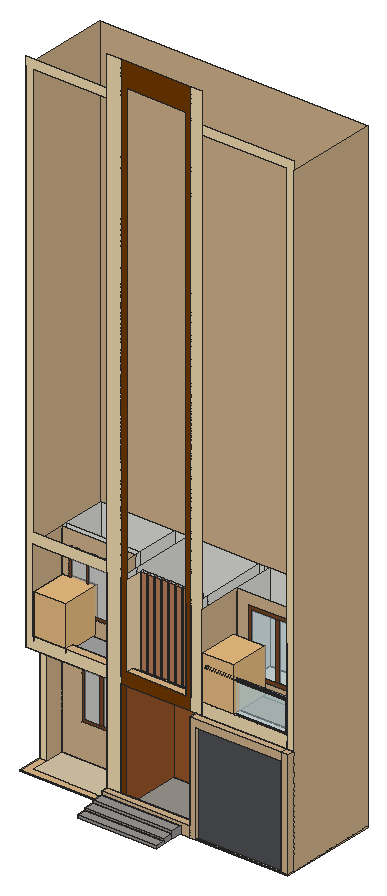
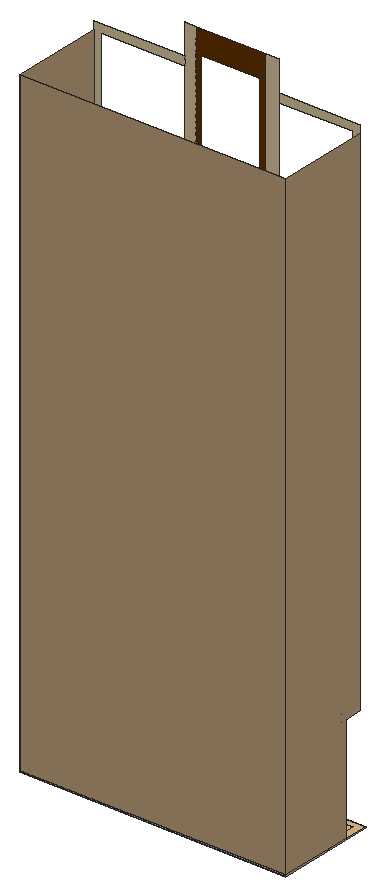
# SketchUp Ruby script. Lengths in inches.
U = 1.inch
M = Sketchup.active_model
def pt(a) = Geom::Point3d.new(a.map { |v| v * U })
def face(e, loops, mat)
  f = e.add_face(loops[0].map { |a| pt(a) })
  loops[1..].each { |l| e.add_face(l.map { |a| pt(a) }).erase! }
  f.material = f.back_material = mat if mat
  f
end
# faces: each face lists its corners as indices into pts; further lists are holes
def faces(e, pts, list, mat = nil) = list.each { |f| face(e, (f[0].is_a?(Array) ? f : [f]).map { |l| l.map { |i| pts[i] } }, mat) }
# xy, xz, yz: faces in a plane at the given z, y or x. An outline is a flat list of corners, or four numbers for a rectangle; further outlines are holes
def ring(l) = l.size == 4 ? [[l[0], l[1]], [l[2], l[1]], [l[2], l[3]], [l[0], l[3]]] : l.each_slice(2).to_a
def flat(e, list, mat, &to3) = list.each { |f| face(e, (f[0].is_a?(Array) ? f : [f]).map { |l| ring(l).map { |u, v| to3.(u, v) } }, mat) }
def xy(e, z, list, mat = nil) = flat(e, list, mat) { |x, y| [x, y, z] }
def xz(e, y, list, mat = nil) = flat(e, list, mat) { |x, z| [x, y, z] }
def yz(e, x, list, mat = nil) = flat(e, list, mat) { |y, z| [x, y, z] }
def lines(e, pts, list) = list.each { |a, b| e.add_line(pt(pts[a]), pt(pts[b])) }
# prism: a flat outline (further loops are holes) pulled along v
def prism(e, loops, v, mat = nil)
  f = face(e, loops, mat); d = Geom::Vector3d.new(v.map { |x| x * U })
  f.pushpull(f.normal.samedirection?(d) ? d.length : -d.length)
end
def box(e, o, s, mat = nil) = prism(e, [[o, [o[0] + s[0], o[1], o[2]], [o[0] + s[0], o[1] + s[1], o[2]], [o[0], o[1] + s[1], o[2]]]], [0, 0, s[2]], mat)
def at(x, y, z, deg = 0) = Geom::Transformation.translation(pt([x, y, z])) * Geom::Transformation.rotation(ORIGIN, Z_AXIS, deg.degrees)
def axes(o, x, y, z) = Geom::Transformation.new([*x, 0, *y, 0, *z, 0, *pt(o).to_a, 1])
def part(name) = M.definitions.add(name)
# library, detail: a bought-in or finely detailed component or shape, given as its bounding box
def library(name, o, s) = part(name).tap { |d| box(d.entities, o, s) }
def detail(e, o, s) = box(e.add_group.entities, o, s)
def put(e, d, t, mat = nil) = e.add_instance(d, t).tap { |i| i.material = mat if mat }
def group(e, t, mat = nil) = e.add_group.tap { |g| g.transformation = t; g.material = mat if mat }.entities
root = M.entities
M.materials.add("[0034_Wheat]").color = [245, 222, 179]
M.materials.add("[0035_Tan]").color = [210, 180, 140]
M.materials.add("[0036_BurlyWood]1").color = [222, 184, 135]
M.materials.add("[Blinds Roman Hobbled Blue]").color = [81, 82, 87]
M.materials.add("[Carpet Berber Pattern Gray]").color = [165, 165, 165]
M.materials.add("[Color C07]").color = [114, 57, 0]
M.materials.add("[Concrete Aggregate Smoke]").color = [154, 150, 148]
M.materials.add("[Field Square Tile]").color = [217, 201, 169]
M.materials.add("[Formica Beige]").color = [247, 219, 174]
M.materials.add("[Formica Laminate Dark]").color = [50, 53, 60]
M.materials.add("[Granite Tile]").color = [155, 148, 143]
M.materials.add("[Tile Veriegated Stone]").color = [171, 137, 112]
M.materials.add("[Translucent Glass Gray]").color = [191, 191, 191]
M.materials["[Translucent Glass Gray]"].alpha = 0.5
M.materials.add("[Translucent Glass Safety]").color = [204, 235, 244]
M.materials["[Translucent Glass Safety]"].alpha = 0.5
M.materials.add("[Wood Cherry Original]1").color = [152, 86, 42]
M.materials.add("[Wood Veneer 01]").color = [120, 70, 37]
M.materials.add("[Wood Veneer 02]").color = [190, 128, 91]
c1 = library("chau cay",[-24.34,-109.24,0],[56.46,62.58,79.69])
xy(root,0,[[646.67,0,1274.49,73.07],[646.67,73.07,1274.49,155.22],[646.67,155.22,1274.49,237.375],[0,237.375,2128.29,1030.11]])
xy(root,9,[[2069.85,237.375,2128.29,295.82],[1398.32,257.25,2069.85,283.5625],[2069.85,295.82,2069.85,971.67,58.44,971.67,58.44,433.5,0,433.5,0,1030.11,2128.29,1030.11,2128.29,295.82],[646.67,295.82,646.67,971.67,726.78,971.67,726.78,763.98,752.97,763.98,752.97,295.82],[752.97,295.82,800.41,763.98],
  [1351.23,295.82,1398.32,971.67],[1398.32,295.82,2069.85,971.67],[58.44,584.29,646.67,971.67],[726.78,763.98,1351.23,971.67]])
xy(root,9,[[0,237.375,646.67,237.375,646.67,295.82,58.44,295.82,58.44,433.5,0,433.5],[1398.32,237.375,2069.85,257.25]],"[0036_BurlyWood]1")
xy(root,9,[[58.44,295.82,646.67,584.29]],"[Field Square Tile]")
xy(root,9,[[800.41,295.82,1351.23,763.98]],"[Granite Tile]")
xy(root,22.375,[[646.67,0,1274.49,73.07]],"[Concrete Aggregate Smoke]")
xy(root,39.375,[[646.67,73.07,1274.49,155.22]],"[Concrete Aggregate Smoke]")
xy(root,58.875,[[646.67,155.22,1274.49,237.375]],"[Concrete Aggregate Smoke]")
xy(root,86.125,[[646.67,237.375,1351.23,295.82]],"[0035_Tan]")
xy(root,800.1875,[[1398.32,237.375,2069.85,257.25]],"[0036_BurlyWood]1")
xy(root,862.75,[[752.97,295.82,800.41,584.29],[1351.23,295.82,1398.32,584.29],[1398.32,295.82,2069.85,584.29],[58.44,584.29,646.67,971.67],[646.67,584.29,646.67,971.67,726.78,971.67,726.78,763.98,752.97,763.98,752.97,584.29],
  [752.97,584.29,800.41,763.98],[1351.23,584.29,1398.32,971.67],[1398.32,584.29,2069.85,971.67],[726.78,763.98,1351.23,971.67]])
xy(root,862.75,[[1351.23,237.375,2069.85,295.82],[2069.85,237.375,2128.29,295.82],[0,295.82,0,433.5,58.44,433.5,58.44,584.29,646.67,584.29,646.67,295.82]],"[0035_Tan]")
xy(root,862.75,[[800.41,295.82,1351.23,584.29],[800.41,584.29,1351.23,763.98]],"[Wood Cherry Original]1")
xy(root,918.8125,[[752.97,358.94,800.41,457.98],[1272.8,358.94,1313.62,457.98],[1313.62,358.94,1398.32,971.67],[800.41,433.79,848.4,457.98],[856.53,433.79,904.52,457.98],
  [912.66,433.79,960.65,457.98],[968.78,433.79,1016.77,457.98],[1024.91,433.79,1072.9,457.98],[1081.03,433.79,1129.02,457.98],[1137.16,433.79,1185.15,457.98],
  [1192.22,433.79,1232.95,457.98],[1240.21,433.79,1272.8,457.98],[752.97,457.98,1313.62,971.67],[58.44,584.29,646.67,623.89],[58.44,623.89,646.67,971.67],
  [1398.32,647.48,2069.85,971.67]])
xy(root,918.8125,[[800.41,358.94,1272.8,358.94,1272.8,433.79,1240.21,433.79,1240.21,457.98,1232.95,457.98,1232.95,433.79,1192.22,433.79,1192.22,457.98,1185.15,457.98,1185.15,433.79,1137.16,433.79,1137.16,457.98,1129.02,457.98,1129.02,433.79,1081.03,433.79,1081.03,457.98,1072.9,457.98,1072.9,433.79,1024.91,433.79,1024.91,457.98,1016.77,457.98,1016.77,433.79,968.78,433.79,968.78,457.98,960.65,457.98,960.65,433.79,912.66,433.79,912.66,457.98,904.52,457.98,904.52,433.79,856.53,433.79,856.53,457.98,848.4,457.98,848.4,433.79,800.41,433.79]],"[0036_BurlyWood]1")
xy(root,918.8125,[[58.44,358.94,646.67,584.29]],"[Carpet Berber Pattern Gray]")
xy(root,918.8125,[[1398.32,358.94,2069.85,647.48]],"[Tile Veriegated Stone]")
xy(root,961.5625,[[1414.96,312.46,2052.74,358.94],[1407.92,319.86,1406.26,319.88,1404.65,320.34,1403.23,321.19,1402.07,322.39,1401.26,323.84,1400.85,325.45,1400.875,327.12,1401.33,328.72,1402.18,330.15,1403.375,331.31,1404.83,332.12,1406.44,332.52,1408.11,332.5,1409.71,332.04,1411.14,331.19,1412.3,330,1413.11,328.54,1413.51,326.93,1413.49,325.27,1413.03,323.66,1412.18,322.24,1410.99,321.08,1409.53,320.27],[2060.17,319.86,2058.51,319.88,2056.9,320.34,2055.48,321.19,2054.32,322.39,2053.51,323.84,2053.1,325.45,2053.125,327.12,2053.58,328.72,2054.43,330.15,2055.625,331.31,2057.08,332.12,2058.69,332.52,2060.36,332.5,2061.96,332.04,2063.39,331.19,2064.55,330,2065.36,328.54,2065.76,326.93,2065.74,325.27,2065.28,323.66,2064.43,322.24,2063.24,321.08,2061.78,320.27]])
xy(root,961.5625,[[1398.32,295.82,2052.74,312.46],[2052.74,295.82,2069.85,312.46],[[1398.32,312.46,1414.96,358.94],[1407.92,319.86,1406.26,319.88,1404.65,320.34,1403.23,321.19,1402.07,322.39,1401.26,323.84,1400.85,325.45,1400.875,327.12,1401.33,328.72,1402.18,330.15,1403.375,331.31,1404.83,332.12,1406.44,332.52,1408.11,332.5,1409.71,332.04,1411.14,331.19,1412.3,330,1413.11,328.54,1413.51,326.93,1413.49,325.27,1413.03,323.66,1412.18,322.24,1410.99,321.08,1409.53,320.27]],[[2052.74,312.46,2069.85,358.94],[2060.17,319.86,2058.51,319.88,2056.9,320.34,2055.48,321.19,2054.32,322.39,2053.51,323.84,2053.1,325.45,2053.125,327.12,2053.58,328.72,2054.43,330.15,2055.625,331.31,2057.08,332.12,2058.69,332.52,2060.36,332.5,2061.96,332.04,2063.39,331.19,2064.55,330,2065.36,328.54,2065.76,326.93,2065.74,325.27,2065.28,323.66,2064.43,322.24,2063.24,321.08,2061.78,320.27]]],"[0034_Wheat]")
xy(root,961.5625,[[58.44,295.82,646.67,358.94],[800.41,295.82,1272.8,358.94]],"[0036_BurlyWood]1")
xy(root,1187.43,[[1414.96,312.46,2052.74,358.94]],"[Translucent Glass Safety]")
xy(root,1192.93,[[1407.92,319.86,1408.5,320.01,1405.82,320.01,1406.26,319.88],[1405.82,320.01,1408.5,320.01,1409.53,320.27,1410.99,321.08,1412.18,322.24,1413.03,323.66,1413.49,325.27,1413.51,326.93,1413.11,328.54,1412.3,330,1411.14,331.19,1409.71,332.04,1408.11,332.5,1406.44,332.52,1404.83,332.12,1403.375,331.31,1402.18,330.15,1401.33,328.72,1400.875,327.12,1400.85,325.45,1401.26,323.84,1402.07,322.39,1403.23,321.19,1404.65,320.34]])
xy(root,1193.4375,[[2060.17,319.86,2061.78,320.27,2063.24,321.08,2064.43,322.24,2065.28,323.66,2065.74,325.27,2065.76,326.93,2065.36,328.54,2064.55,330,2063.39,331.19,2061.96,332.04,2060.36,332.5,2058.69,332.52,2057.08,332.12,2055.625,331.31,2054.43,330.15,2053.58,328.72,2053.125,327.12,2053.1,325.45,2053.51,323.84,2054.32,322.39,2055.48,321.19,2056.9,320.34,2058.51,319.88]])
xz(root,0,[[646.67,0,1274.49,22.375]],"[Concrete Aggregate Smoke]")
xz(root,73.07,[[646.67,0,1274.49,22.375]])
xz(root,73.07,[[646.67,22.375,1274.49,39.375]],"[Concrete Aggregate Smoke]")
xz(root,155.22,[[646.67,0,1274.49,39.375]])
xz(root,155.22,[[646.67,39.375,1274.49,58.875]],"[Concrete Aggregate Smoke]")
xz(root,237.375,[[646.67,0,1274.49,58.875]])
xz(root,237.375,[[1274.49,0,1351.23,0,1351.23,86.125,646.67,86.125,646.67,58.875,1274.49,58.875],[1351.23,0,1398.32,0,1398.32,800.1875,2069.85,800.1875,2069.85,862.75,1351.23,862.75],[2069.85,9,2128.29,862.75]],"[0035_Tan]")
xz(root,237.375,[[0,0,646.67,9],[1398.32,0,2128.29,9]],"[0036_BurlyWood]1")
xz(root,257.25,[[1398.32,9,2069.85,800.1875]],"[Blinds Roman Hobbled Blue]")
xz(root,295.82,[[646.67,9,752.97,86.125],[752.97,9,800.41,86.125],[1351.23,9,1398.32,862.75],[1398.32,9,2069.85,862.75],[2069.85,9,2128.29,862.75]])
xz(root,295.82,[[646.67,86.125,752.97,5306.25],[0,862.75,646.67,862.75,646.67,961.5625,58.44,961.5625,58.44,1615.875,646.67,1615.875,646.67,1695.75,58.44,1695.75,58.44,4996.25,646.67,4996.25,646.67,5063.875,0,5063.875],[1313.62,862.75,1398.32,5306.25],[1398.32,862.75,2069.85,961.5625],[2069.85,862.75,2128.29,862.75,2128.29,5063.875,1398.32,5063.875,1398.32,4996.25,2069.85,4996.25]],"[0034_Wheat]")
xz(root,295.82,[[800.41,9,1351.23,86.125]],"[0035_Tan]")
xz(root,295.82,[[752.97,86.125,800.41,862.75],[[752.97,862.75,1313.62,5306.25],[800.41,961.5625,1272.8,5116.2]]],"[Color C07]")
xz(root,312.46,[[1414.96,961.5625,2052.74,1187.43]],"[Translucent Glass Safety]")
xz(root,358.94,[[58.44,918.8125,646.67,961.5625],[1272.8,918.8125,1313.62,961.5625],[1313.62,918.8125,1398.32,961.5625],[1398.32,918.8125,2069.85,961.5625]])
xz(root,358.94,[[800.41,918.8125,1272.8,961.5625]],"[0036_BurlyWood]1")
xz(root,358.94,[[1414.96,961.5625,2052.74,1187.43]],"[Translucent Glass Safety]")
xz(root,433.5,[[0,9,58.44,862.75]],"[0034_Wheat]")
xz(root,433.79,[[800.41,918.8125,848.4,1615.875],[856.53,918.8125,904.52,1615.875],[912.66,918.8125,960.65,1615.875],[968.78,918.8125,1016.77,1615.875],[1024.91,918.8125,1072.9,1615.875],
  [1081.03,918.8125,1129.02,1615.875],[1137.16,918.8125,1185.15,1615.875],[1192.22,918.8125,1232.95,1615.875],[1240.21,918.8125,1272.8,1615.875]],"[Wood Veneer 02]")
xz(root,457.98,[[800.41,918.8125,848.4,1615.875],[856.53,918.8125,904.52,1615.875],[912.66,918.8125,960.65,1615.875],[968.78,918.8125,1016.77,1615.875],[1024.91,918.8125,1072.9,1615.875],
  [1081.03,918.8125,1129.02,1615.875],[1137.16,918.8125,1185.15,1615.875],[1192.22,918.8125,1232.95,1615.875],[1240.21,918.8125,1272.8,1615.875]])
xz(root,457.98,[[848.4,918.8125,856.53,1615.875],[904.52,918.8125,912.66,1615.875],[960.65,918.8125,968.78,1615.875],[1016.77,918.8125,1024.91,1615.875],[1072.9,918.8125,1081.03,1615.875],
  [1129.02,918.8125,1137.16,1615.875],[1185.15,918.8125,1192.22,1615.875],[1232.95,918.8125,1240.21,1615.875]],"[Formica Laminate Dark]")
xz(root,584.29,[[[58.44,9,646.67,862.75],[211.5625,275.46,542.4375,741.34]],[[58.44,918.8125,646.67,1615.875],[113.6,1037.93,575.6,1499.93]]],"[0035_Tan]")
xz(root,584.29,[[234.18,298.08,360.07,718.72],[385.8125,298.08,519.82,718.72],[133.43,1057.76,252.99,1480.1],[266.84,1057.76,428.61,1480.1],[442.47,1057.76,555.77,1480.1]],"[Translucent Glass Gray]")
xz(root,584.29,[[[211.5625,275.46,542.4375,741.34],[234.18,298.08,519.82,718.72]],[360.07,298.08,385.8125,718.72],[[113.6,1037.93,575.6,1499.93],[133.43,1057.76,555.77,1480.1]],[252.99,1057.76,266.84,1480.1],[428.61,1057.76,442.47,1480.1]],"[Wood Veneer 01]")
xz(root,623.89,[[58.44,918.8125,646.67,1615.875]])
xz(root,647.48,[[[1398.32,918.8125,2069.85,1615.875],[1485.05,1017.34,1964.11,1534.78]]],"[0035_Tan]")
xz(root,647.48,[[1515.31,1047.6,1702.55,1504.52],[1732.8,1047.6,1933.85,1504.52]],"[Translucent Glass Safety]")
xz(root,647.48,[[[1485.05,1017.34,1964.11,1534.78],[1515.31,1047.6,1933.85,1504.52]],[1702.55,1047.6,1732.8,1504.52]],"[Wood Veneer 01]")
xz(root,763.98,[[726.78,9,752.97,862.75],[752.97,9,800.41,862.75]])
xz(root,763.98,[[800.41,9,1351.23,862.75]],"[Wood Cherry Original]1")
xz(root,971.67,[[58.44,9,646.67,862.75],[646.67,9,726.78,862.75],[726.78,9,1351.23,862.75],[1351.23,9,1398.32,862.75],[1398.32,9,2069.85,862.75],
  [58.44,862.75,646.67,918.8125],[646.67,862.75,726.78,918.8125],[726.78,862.75,1351.23,918.8125],[1351.23,862.75,1398.32,918.8125],[1398.32,862.75,2069.85,918.8125],
  [58.44,918.8125,646.67,1615.875],[646.67,918.8125,726.78,1615.875],[726.78,918.8125,752.97,1615.875],[752.97,918.8125,1313.62,1615.875],[1313.62,918.8125,1351.23,1615.875],
  [1351.23,918.8125,1398.32,1615.875],[1398.32,918.8125,2069.85,1615.875]])
xz(root,1030.11,[[0,0,2128.29,9]])
xz(root,1030.11,[[0,9,2128.29,4996.25]],"[0035_Tan]")
yz(root,0,[[433.5,9,433.5,862.75,295.82,862.75,295.82,4996.25,1030.11,4996.25,1030.11,9]],"[0035_Tan]")
yz(root,0,[[237.375,0,1030.11,9]],"[0036_BurlyWood]1")
yz(root,58.44,[[584.29,9,971.67,862.75],[481.57,862.75,584.29,918.8125],[584.29,862.75,971.67,918.8125],[584.29,918.8125,623.89,1615.875],[623.89,918.8125,971.67,1615.875]])
yz(root,58.44,[[433.5,9,584.29,862.75],[358.94,918.8125,584.29,918.8125,584.29,1615.875,295.82,1615.875,295.82,961.5625,358.94,961.5625]],"[0035_Tan]")
yz(root,646.67,[[584.29,9,971.67,862.75],[295.82,862.75,971.67,918.8125],[295.82,918.8125,358.94,961.5625],[584.29,918.8125,623.89,1615.875],[623.89,918.8125,971.67,1615.875]])
yz(root,646.67,[[295.82,9,584.29,862.75],[358.94,918.8125,358.94,961.5625,295.82,961.5625,295.82,1615.875,584.29,1615.875,584.29,918.8125]],"[0035_Tan]")
yz(root,646.67,[[237.375,9,295.82,86.125]],"[0036_BurlyWood]1")
yz(root,646.67,[[0,0,73.07,22.375],[73.07,0,155.22,39.375],[155.22,0,237.375,58.875]],"[Concrete Aggregate Smoke]")
yz(root,726.78,[[763.98,9,971.67,862.75]])
yz(root,752.97,[[295.82,9,763.98,862.75],[295.82,918.8125,457.98,1615.875],[457.98,918.8125,971.67,1615.875]])
yz(root,800.41,[[433.79,918.8125,457.98,1615.875]])
yz(root,800.41,[[358.94,918.8125,433.79,918.8125,433.79,1615.875,295.82,1615.875,295.82,961.5625,358.94,961.5625]],"[Formica Beige]")
yz(root,800.41,[[295.82,9,763.98,862.75]],"[Wood Cherry Original]1")
yz(root,848.4,[[433.79,918.8125,457.98,1615.875]],"[Wood Veneer 02]")
yz(root,856.53,[[433.79,918.8125,457.98,1615.875]],"[Wood Veneer 02]")
yz(root,904.52,[[433.79,918.8125,457.98,1615.875]],"[Wood Veneer 02]")
yz(root,912.66,[[433.79,918.8125,457.98,1615.875]],"[Wood Veneer 02]")
yz(root,960.65,[[433.79,918.8125,457.98,1615.875]],"[Wood Veneer 02]")
yz(root,968.78,[[433.79,918.8125,457.98,1615.875]],"[Wood Veneer 02]")
yz(root,1016.77,[[433.79,918.8125,457.98,1615.875]],"[Wood Veneer 02]")
yz(root,1024.91,[[433.79,918.8125,457.98,1615.875]],"[Wood Veneer 02]")
yz(root,1072.9,[[433.79,918.8125,457.98,1615.875]],"[Wood Veneer 02]")
yz(root,1081.03,[[433.79,918.8125,457.98,1615.875]],"[Wood Veneer 02]")
yz(root,1129.02,[[433.79,918.8125,457.98,1615.875]],"[Wood Veneer 02]")
yz(root,1137.16,[[433.79,918.8125,457.98,1615.875]],"[Wood Veneer 02]")
yz(root,1185.15,[[433.79,918.8125,457.98,1615.875]],"[Wood Veneer 02]")
yz(root,1192.22,[[433.79,918.8125,457.98,1615.875]],"[Wood Veneer 02]")
yz(root,1232.95,[[433.79,918.8125,457.98,1615.875]],"[Wood Veneer 02]")
yz(root,1240.21,[[433.79,918.8125,457.98,1615.875]],"[Wood Veneer 02]")
yz(root,1272.8,[[433.79,918.8125,457.98,1615.875]])
yz(root,1272.8,[[358.94,918.8125,358.94,961.5625,295.82,961.5625,295.82,1615.875,433.79,1615.875,433.79,918.8125]],"[Formica Beige]")
yz(root,1274.49,[[0,0,73.07,22.375],[73.07,0,155.22,39.375],[155.22,0,237.375,58.875]],"[Concrete Aggregate Smoke]")
yz(root,1313.62,[[358.94,918.8125,457.98,918.8125,457.98,1615.875,295.82,1615.875,295.82,961.5625,358.94,961.5625],[457.98,918.8125,971.67,1615.875]])
yz(root,1351.23,[[763.98,9,971.67,862.75]])
yz(root,1351.23,[[237.375,86.125,295.82,862.75]],"[0035_Tan]")
yz(root,1351.23,[[295.82,9,763.98,862.75]],"[Wood Cherry Original]1")
yz(root,1398.32,[[295.82,9,971.67,862.75],[295.82,862.75,971.67,918.8125],[295.82,918.8125,358.94,961.5625],[647.48,918.8125,971.67,1615.875]])
yz(root,1398.32,[[237.375,9,257.25,800.1875],[[358.94,918.8125,647.48,918.8125,647.48,1615.875,295.82,1615.875,295.82,961.5625,358.94,961.5625],[327.38,1185.55,325.47,1185.8,323.69,1186.54,322.17,1187.71,320.99,1189.24,320.26,1191.02,320.01,1192.93,320.26,1194.84,320.99,1196.62,322.17,1198.14,323.69,1199.32,325.47,1200.05,327.38,1200.3,329.29,1200.05,331.07,1199.32,332.6,1198.14,333.77,1196.62,334.5,1194.84,334.76,1192.93,334.5,1191.02,333.77,1189.24,332.6,1187.71,331.07,1186.54,329.29,1185.8]]],"[0035_Tan]")
yz(root,1414.96,[[312.46,961.5625,358.94,1187.43]])
yz(root,2052.74,[[312.46,961.5625,358.94,1187.43]])
yz(root,2069.85,[[257.25,9,283.5625,800.1875],[295.82,9,971.67,862.75],[295.82,862.75,481.57,918.8125],[481.57,862.75,584.29,918.8125],[584.29,862.75,971.67,918.8125],
  [647.48,918.8125,971.67,1615.875],[327.38,1185.55,329.29,1185.8,331.07,1186.54,332.6,1187.71,333.77,1189.24,334.5,1191.02,334.76,1192.93,334.5,1194.84,333.77,1196.62,332.6,1198.14,331.07,1199.32,329.29,1200.05,327.38,1200.3,325.47,1200.05,323.69,1199.32,322.17,1198.14,320.99,1196.62,320.26,1194.84,320.01,1192.93,320.26,1191.02,320.99,1189.24,322.17,1187.71,323.69,1186.54,325.47,1185.8]])
yz(root,2069.85,[[237.375,9,257.25,800.1875],[[358.94,918.8125,358.94,961.5625,295.82,961.5625,295.82,1615.875,647.48,1615.875,647.48,918.8125],[327.38,1185.55,329.29,1185.8,331.07,1186.54,332.6,1187.71,333.77,1189.24,334.5,1191.02,334.76,1192.93,334.5,1194.84,333.77,1196.62,332.6,1198.14,331.07,1199.32,329.29,1200.05,327.38,1200.3,325.47,1200.05,323.69,1199.32,322.17,1198.14,320.99,1196.62,320.26,1194.84,320.01,1192.93,320.26,1191.02,320.99,1189.24,322.17,1187.71,323.69,1186.54,325.47,1185.8]]],"[0035_Tan]")
yz(root,2128.29,[[237.375,9,295.82,862.75],[295.82,9,1030.11,4996.25]],"[0035_Tan]")
yz(root,2128.29,[[237.375,0,1030.11,9]],"[0036_BurlyWood]1")
p = [[1404.65,320.34,961.5625],[1406.26,319.88,961.5625],[1406.26,319.88,1192.93],[1405.82,320.01,1192.93],[1404.65,320.34,1192.93],[1407.92,319.86,961.5625],
  [1407.92,319.86,1192.93],[1409.53,320.27,961.5625],[1409.53,320.27,1192.93],[1408.5,320.01,1192.93],[2056.9,320.34,961.5625],[2058.51,319.88,961.5625],
  [2058.51,319.88,1193.4375],[2056.9,320.34,1193.4375],[2060.17,319.86,961.5625],[2060.17,319.86,1193.4375],[2061.78,320.27,961.5625],[2061.78,320.27,1193.4375],
  [1403.23,321.19,961.5625],[1403.23,321.19,1192.93],[1410.99,321.08,961.5625],[1410.99,321.08,1192.93],[2055.48,321.19,961.5625],[2055.48,321.19,1193.4375],
  [2063.24,321.08,961.5625],[2063.24,321.08,1193.4375],[1412.18,322.24,961.5625],[1412.18,322.24,1192.93],[2064.43,322.24,961.5625],[2064.43,322.24,1193.4375],
  [1402.07,322.39,961.5625],[1402.07,322.39,1192.93],[2054.32,322.39,961.5625],[2054.32,322.39,1193.4375],[1413.03,323.66,961.5625],[1413.03,323.66,1192.93],
  [2065.28,323.66,961.5625],[2065.28,323.66,1193.4375],[1401.26,323.84,961.5625],[1401.26,323.84,1192.93],[2053.51,323.84,961.5625],[2053.51,323.84,1193.4375],
  [1413.49,325.27,961.5625],[1413.49,325.27,1192.93],[2065.74,325.27,961.5625],[2065.74,325.27,1193.4375],[1400.85,325.45,961.5625],[1400.85,325.45,1192.93],
  [2053.1,325.45,961.5625],[2053.1,325.45,1193.4375],[1413.51,326.93,961.5625],[1413.51,326.93,1192.93],[2065.76,326.93,961.5625],[2065.76,326.93,1193.4375],
  [1400.875,327.12,961.5625],[1400.875,327.12,1192.93],[2053.125,327.12,961.5625],[2053.125,327.12,1193.4375],[1413.11,328.54,961.5625],[1413.11,328.54,1192.93],
  [2065.36,328.54,961.5625],[2065.36,328.54,1193.4375],[1401.33,328.72,961.5625],[1401.33,328.72,1192.93],[2053.58,328.72,961.5625],[2053.58,328.72,1193.4375],
  [1412.3,330,961.5625],[1412.3,330,1192.93],[2064.55,330,961.5625],[2064.55,330,1193.4375],[1402.18,330.15,961.5625],[1402.18,330.15,1192.93],
  [2054.43,330.15,961.5625],[2054.43,330.15,1193.4375],[1411.14,331.19,961.5625],[1411.14,331.19,1192.93],[2063.39,331.19,961.5625],[2063.39,331.19,1193.4375],
  [1403.375,331.31,961.5625],[1403.375,331.31,1192.93],[2055.625,331.31,961.5625],[2055.625,331.31,1193.4375],[1409.71,332.04,961.5625],[1409.71,332.04,1192.93],
  [2061.96,332.04,961.5625],[2061.96,332.04,1193.4375],[1404.83,332.12,961.5625],[1404.83,332.12,1192.93],[2057.08,332.12,961.5625],[2057.08,332.12,1193.4375],
  [1408.11,332.5,961.5625],[1408.11,332.5,1192.93],[2060.36,332.5,961.5625],[2060.36,332.5,1193.4375],[1406.44,332.52,961.5625],[1406.44,332.52,1192.93],
  [2058.69,332.52,961.5625],[2058.69,332.52,1193.4375],[2069.85,327.38,1185.55],[2069.85,325.47,1185.8],[1398.32,325.47,1185.8],[1398.32,327.38,1185.55],
  [2069.85,329.29,1185.8],[1398.32,329.29,1185.8],[2069.85,323.69,1186.54],[1398.32,323.69,1186.54],[2069.85,331.07,1186.54],[1398.32,331.07,1186.54],
  [2069.85,322.17,1187.71],[1398.32,322.17,1187.71],[2069.85,332.6,1187.71],[1398.32,332.6,1187.71],[2069.85,320.99,1189.24],[1398.32,320.99,1189.24],
  [2069.85,333.77,1189.24],[1398.32,333.77,1189.24],[2069.85,320.26,1191.02],[1398.32,320.26,1191.02],[2069.85,334.5,1191.02],[1398.32,334.5,1191.02],
  [2069.85,320.01,1192.93],[1398.32,320.01,1192.93],[2069.85,334.76,1192.93],[1398.32,334.76,1192.93],[2069.85,320.26,1194.84],[1398.32,320.26,1194.84],
  [2069.85,334.5,1194.84],[1398.32,334.5,1194.84],[2069.85,320.99,1196.62],[1398.32,320.99,1196.62],[2069.85,333.77,1196.62],[1398.32,333.77,1196.62],
  [2069.85,322.17,1198.14],[1398.32,322.17,1198.14],[2069.85,332.6,1198.14],[1398.32,332.6,1198.14],[2069.85,323.69,1199.32],[1398.32,323.69,1199.32],
  [2069.85,331.07,1199.32],[1398.32,331.07,1199.32],[2069.85,325.47,1200.05],[1398.32,325.47,1200.05],[2069.85,329.29,1200.05],[1398.32,329.29,1200.05],
  [2069.85,327.38,1200.3],[1398.32,327.38,1200.3],[58.44,481.57,918.8125],[0,481.57,918.8125],[58.44,481.57,862.75],[0,481.57,862.75],
  [58.44,358.94,918.8125],[58.44,295.82,918.8125],[800.41,358.94,918.8125],[800.41,295.82,918.8125]]
faces(root,p,[[0,1,2,3,4],[1,5,6,2],[5,7,8,9,6],[10,11,12,13],[11,14,15,12],[14,16,17,15],[18,0,4,19],[7,20,21,8],
  [22,10,13,23],[16,24,25,17],[20,26,27,21],[24,28,29,25],[30,18,19,31],[32,22,23,33],[26,34,35,27],[28,36,37,29],
  [38,30,31,39],[40,32,33,41],[34,42,43,35],[36,44,45,37],[46,38,39,47],[48,40,41,49],[42,50,51,43],[44,52,53,45],
  [54,46,47,55],[56,48,49,57],[50,58,59,51],[52,60,61,53],[62,54,55,63],[64,56,57,65],[58,66,67,59],[60,68,69,61],
  [70,62,63,71],[72,64,65,73],[66,74,75,67],[68,76,77,69],[78,70,71,79],[80,72,73,81],[74,82,83,75],[76,84,85,77],
  [86,78,79,87],[88,80,81,89],[82,90,91,83],[84,92,93,85],[94,86,87,95],[96,88,89,97],[90,94,95,91],[92,96,97,93],
  [98,99,100,101],[102,98,101,103],[99,104,105,100],[106,102,103,107],[104,108,109,105],[110,106,107,111],[108,112,113,109],[114,110,111,115],
  [112,116,117,113],[118,114,115,119],[116,120,9,3,121,117],[122,118,119,123],[120,124,125,121,3,9],[126,122,123,127],[124,128,129,125],[130,126,127,131],
  [128,132,133,129],[134,130,131,135],[132,136,137,133],[138,134,135,139],[136,140,141,137],[142,138,139,143],[140,144,145,141],[144,142,143,145]],"[Formica Laminate Dark]")
lines(root,p,[[146,147],[148,149],[150,151],[152,153]])
put(root,c1,axes([169.76,64.16,926.125],[4.5,0,0],[0,-4.9651,0],[0,0,4.37432]))
put(root,c1,axes([1507.85,64.16,961.5625],[4.5,0,0],[0,-4.9651,0],[0,0,4.37432]))
